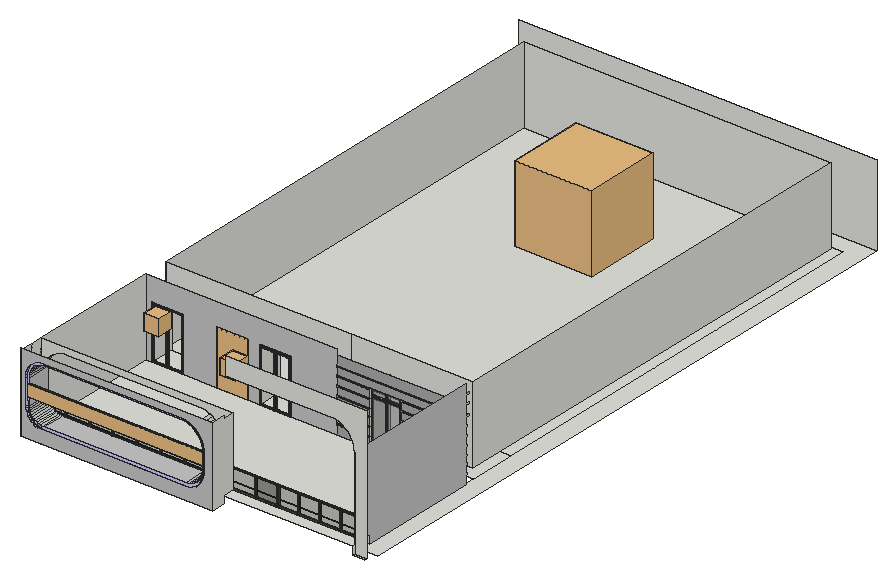
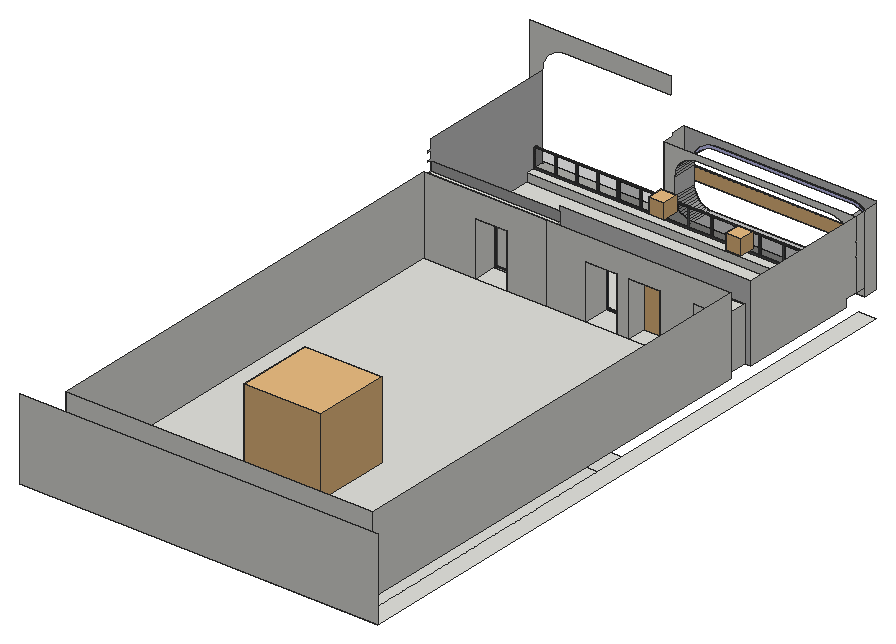
# SketchUp Ruby script. Lengths in inches.
U = 1.inch
M = Sketchup.active_model
def pt(a) = Geom::Point3d.new(a.map { |v| v * U })
def face(e, loops, mat)
  f = e.add_face(loops[0].map { |a| pt(a) })
  loops[1..].each { |l| e.add_face(l.map { |a| pt(a) }).erase! }
  f.material = f.back_material = mat if mat
  f
end
# faces: each face lists its corners as indices into pts; further lists are holes
def faces(e, pts, list, mat = nil) = list.each { |f| face(e, (f[0].is_a?(Array) ? f : [f]).map { |l| l.map { |i| pts[i] } }, mat) }
# xy, xz, yz: faces in a plane at the given z, y or x. An outline is a flat list of corners, or four numbers for a rectangle; further outlines are holes
def ring(l) = l.size == 4 ? [[l[0], l[1]], [l[2], l[1]], [l[2], l[3]], [l[0], l[3]]] : l.each_slice(2).to_a
def flat(e, list, mat, &to3) = list.each { |f| face(e, (f[0].is_a?(Array) ? f : [f]).map { |l| ring(l).map { |u, v| to3.(u, v) } }, mat) }
def xy(e, z, list, mat = nil) = flat(e, list, mat) { |x, y| [x, y, z] }
def xz(e, y, list, mat = nil) = flat(e, list, mat) { |x, z| [x, y, z] }
def yz(e, x, list, mat = nil) = flat(e, list, mat) { |y, z| [x, y, z] }
def lines(e, pts, list) = list.each { |a, b| e.add_line(pt(pts[a]), pt(pts[b])) }
# prism: a flat outline (further loops are holes) pulled along v
def prism(e, loops, v, mat = nil)
  f = face(e, loops, mat); d = Geom::Vector3d.new(v.map { |x| x * U })
  f.pushpull(f.normal.samedirection?(d) ? d.length : -d.length)
end
def box(e, o, s, mat = nil) = prism(e, [[o, [o[0] + s[0], o[1], o[2]], [o[0] + s[0], o[1] + s[1], o[2]], [o[0], o[1] + s[1], o[2]]]], [0, 0, s[2]], mat)
def at(x, y, z, deg = 0) = Geom::Transformation.translation(pt([x, y, z])) * Geom::Transformation.rotation(ORIGIN, Z_AXIS, deg.degrees)
def axes(o, x, y, z) = Geom::Transformation.new([*x, 0, *y, 0, *z, 0, *pt(o).to_a, 1])
def part(name) = M.definitions.add(name)
# library, detail: a bought-in or finely detailed component or shape, given as its bounding box
def library(name, o, s) = part(name).tap { |d| box(d.entities, o, s) }
def detail(e, o, s) = box(e.add_group.entities, o, s)
def put(e, d, t, mat = nil) = e.add_instance(d, t).tap { |i| i.material = mat if mat }
def group(e, t, mat = nil) = e.add_group.tap { |g| g.transformation = t; g.material = mat if mat }.entities
root = M.entities
M.materials.add("Aluminum_Polished").color = [83, 85, 85]
M.materials.add("Glass_Window_Neutral").color = [0, 0, 0]
M.materials["Glass_Window_Neutral"].alpha = 0.125
M.materials.add("Wine2").color = [0, 0, 0]
M.materials["Wine2"].alpha = 0
M.materials.add("[0130_Gainsboro]").color = [39, 45, 50]
M.materials.add("[Color I01]").color = [204, 204, 255]
M.materials.add("[Color M02]").color = [198, 198, 198]
M.materials.add("[Color M03]").color = [170, 170, 170]
M.materials.add("[Color M06]").color = [86, 86, 86]
M.materials.add("[Translucent Glass Gray]").color = [128, 128, 128]
M.materials["[Translucent Glass Gray]"].alpha = 0.5
c1 = part("Framed glazing panel")
xy(c1.entities,0,[[0,-0.98,43.07,0],[0,0,43.07,1.4]],"[0130_Gainsboro]")
xy(c1.entities,0.3,[[0.3,-1.43,42.77,-0.98]],"[0130_Gainsboro]")
xy(c1.entities,2.95,[[2.95,-1.43,40.12,-0.63],[2.95,-0.63,40.12,0],[2.95,0,40.12,0.64],[2.95,0.64,40.12,1.4]],"[0130_Gainsboro]")
xy(c1.entities,3.54,[[3.54,-0.63,39.53,0],[3.54,0,39.53,0.64]],"[0130_Gainsboro]")
xy(c1.entities,111.8125,[[3.54,-0.63,39.53,0],[3.54,0,39.53,0.64]],"[0130_Gainsboro]")
xy(c1.entities,112.4,[[2.95,-1.43,40.12,-0.63],[2.95,-0.63,40.12,0],[2.95,0,40.12,0.64],[2.95,0.64,40.12,1.4]],"[0130_Gainsboro]")
xy(c1.entities,115.05,[[0.3,-1.43,42.77,-0.98]],"[0130_Gainsboro]")
xy(c1.entities,115.35,[[0,-0.98,43.07,0],[0,0,43.07,1.4]],"[0130_Gainsboro]")
xz(c1.entities,-1.43,[[[0.3,0.3,42.77,115.05],[2.95,2.95,40.12,112.4]]],"[0130_Gainsboro]")
xz(c1.entities,-0.98,[[[0,0,43.07,115.35],[0.3,0.3,42.77,115.05]]],"[0130_Gainsboro]")
xz(c1.entities,-0.63,[[[2.95,2.95,40.12,112.4],[3.54,3.54,39.53,111.8125]]],"[0130_Gainsboro]")
xz(c1.entities,0,[[3.54,3.54,39.53,111.8125]],"Wine2")
xz(c1.entities,0,[[[0,0,43.07,115.35],[2.95,2.95,40.12,112.4]],[[2.95,2.95,40.12,112.4],[3.54,3.54,39.53,111.8125]]],"[0130_Gainsboro]")
xz(c1.entities,0.64,[[[2.95,2.95,40.12,112.4],[3.54,3.54,39.53,111.8125]]],"[0130_Gainsboro]")
xz(c1.entities,1.4,[[[0,0,43.07,115.35],[2.95,2.95,40.12,112.4]]],"[0130_Gainsboro]")
yz(c1.entities,0,[[-0.98,0,0,115.35],[0,0,1.4,115.35]],"[0130_Gainsboro]")
yz(c1.entities,0.3,[[-1.43,0.3,-0.98,115.05]],"[0130_Gainsboro]")
yz(c1.entities,2.95,[[-1.43,2.95,-0.63,112.4],[-0.63,2.95,0,112.4],[0,2.95,0.64,112.4],[0.64,2.95,1.4,112.4]],"[0130_Gainsboro]")
yz(c1.entities,3.54,[[-0.63,3.54,0,111.8125],[0,3.54,0.64,111.8125]],"[0130_Gainsboro]")
yz(c1.entities,39.53,[[-0.63,3.54,0,111.8125],[0,3.54,0.64,111.8125]],"[0130_Gainsboro]")
yz(c1.entities,40.12,[[-1.43,2.95,-0.63,112.4],[-0.63,2.95,0,112.4],[0,2.95,0.64,112.4],[0.64,2.95,1.4,112.4]],"[0130_Gainsboro]")
yz(c1.entities,42.77,[[-1.43,0.3,-0.98,115.05]],"[0130_Gainsboro]")
yz(c1.entities,43.07,[[-0.98,0,0,115.35],[0,0,1.4,115.35]],"[0130_Gainsboro]")
c2 = part("Group\#1")
put(c2.entities,c1,axes([45.29,1.43,0],[1.05148,0,0],[0,1,0],[0,0,1]))
put(c2.entities,c1,axes([0,1.43,0],[1.05148,0,0],[0,1,0],[0,0,1]))
c3 = library("door (1)",[38.93,25.48,0],[40,9.94,82.68])
c4 = part("Group\#3")
xy(c4.entities,0,[[0,0,32.48,1.97]])
xy(c4.entities,0.98,[[0.98,0,31.5,0.98],[0.98,0.98,31.5,1.97]])
xy(c4.entities,8.86,[[0.98,0,31.5,0.98],[0.98,0.98,31.5,1.97]])
xy(c4.entities,9.84,[[0,0,32.48,1.97]])
xz(c4.entities,0,[[[0,0,32.48,9.84],[0.98,0.98,31.5,8.86]]])
xz(c4.entities,0.98,[[0.98,0.98,31.5,8.86]],"[Translucent Glass Gray]")
xz(c4.entities,1.97,[[[0,0,32.48,9.84],[0.98,0.98,31.5,8.86]]])
yz(c4.entities,0,[[0,0,1.97,9.84]])
yz(c4.entities,0.98,[[0,0.98,0.98,8.86],[0.98,0.98,1.97,8.86]])
yz(c4.entities,31.5,[[0,0.98,0.98,8.86],[0.98,0.98,1.97,8.86]])
yz(c4.entities,32.48,[[0,0,1.97,9.84]])
c5 = part("Group\#4")
xy(c5.entities,0,[[0,0,32.48,1.97]])
xy(c5.entities,0.98,[[0.98,0,31.5,0.98],[0.98,0.98,31.5,1.97]])
xy(c5.entities,71.85,[[0.98,0,31.5,0.98],[0.98,0.98,31.5,1.97]])
xy(c5.entities,72.83,[[0,0,32.48,1.97]])
xz(c5.entities,0,[[[0,0,32.48,72.83],[0.98,0.98,31.5,71.85]]])
xz(c5.entities,0.98,[[0.98,0.98,31.5,71.85]],"[Translucent Glass Gray]")
xz(c5.entities,1.97,[[[0,0,32.48,72.83],[0.98,0.98,31.5,71.85]]])
yz(c5.entities,0,[[0,0,1.97,72.83]])
yz(c5.entities,0.98,[[0,0.98,0.98,71.85],[0.98,0.98,1.97,71.85]])
yz(c5.entities,31.5,[[0,0.98,0.98,71.85],[0.98,0.98,1.97,71.85]])
yz(c5.entities,32.48,[[0,0,1.97,72.83]])
c6 = part("FIXED+GLASS+WINDOW+WITH+TRANSOM")
g1 = group(c6.entities,at(0,0,0))
xy(g1,0,[[0,0,70.86,3.9375]])
xy(g1,1.97,[[1.97,0,34.45,0.98],[36.42,0,68.9,3.9375],[1.97,2.95,34.45,3.9375]])
xy(g1,86.61,[[1.97,0,34.45,3.9375],[34.45,0,36.42,3.9375],[36.42,0,68.9,3.9375]])
xy(g1,88.58,[[0,0,70.86,3.9375]])
xz(g1,0,[[[0,0,70.86,88.58],[1.97,1.97,34.45,86.61],[36.42,1.97,68.9,86.61]]])
xz(g1,3.9375,[[[0,0,70.86,88.58],[1.97,1.97,34.45,86.61],[36.42,1.97,68.9,86.61]]])
yz(g1,0,[[0,0,3.9375,88.58]])
yz(g1,1.97,[[0,1.97,3.9375,74.8],[0,76.77,3.9375,86.61]])
yz(g1,34.45,[[0,1.97,3.9375,86.61]])
yz(g1,36.42,[[0,1.97,3.9375,86.61]])
yz(g1,68.9,[[0,1.97,3.9375,86.61]])
yz(g1,70.86,[[0,0,3.9375,88.58]])
g2 = group(g1,at(1.97,0,74.8))
box(g2,[0,0,0],[66.93,3.9375,1.97])
put(g1,c4,at(1.97,0.98,76.77))
put(g1,c4,at(36.42,0.98,76.77))
put(g1,c5,at(1.97,0.98,1.97))
put(g1,c5,at(36.42,0.98,1.97))
c7 = library("Omni Light",[-12,-12,-12],[24,24,24])
c8 = part("Group\#54")
box(c8.entities,[0,0,0],[2,1,28])
c9 = part("Group\#56")
p = [[0.11,0.32,0.14],[0.11,0.69,0.14]]
lines(c9.entities,p,[[0,1]])
g3 = group(c9.entities,at(0.11,0,0))
prism(g3,[[[0,0.24,0],[0,0.32,0.14],[0,0.24,0.27],[0,0.08,0.27],[0,0,0.14],[0,0.08,0]]],[-0.11,0,0])
c10 = part("Ver Glass Railing")
g4 = group(c10.entities,at(0,0,0),"Aluminum_Polished")
box(g4,[0,0,0],[2,185,2])
g5 = group(c10.entities,at(0,0,2),"Aluminum_Polished")
p = [[1.41,1,0],[1.41,36.8,0],[1.41,184,0],[1.29,184,0],[1.29,1,0],[1.29,36.8,0],
  [1.41,184,28],[1.29,184,28],[1.41,148.2,28],[1.29,148.2,28],[1.41,1,28],[1.29,1,28],
  [1.29,111.4,28],[1.29,111.4,0],[1.41,111.4,0],[1.41,111.4,28],[1.29,110.4,0],[1.29,110.4,28],
  [1.41,110.4,28],[1.41,110.4,0],[1.29,74.6,28],[1.29,74.6,0],[1.41,74.6,0],[1.41,74.6,28],
  [1.29,73.6,0],[1.29,73.6,28],[1.41,73.6,28],[1.41,73.6,0],[1.29,148.2,0],[1.41,148.2,0],
  [1.29,147.2,0],[1.29,147.2,28],[1.41,147.2,28],[1.41,147.2,0],[1.29,37.8,28],[1.29,37.8,0],
  [1.41,37.8,0],[1.41,37.8,28],[1.29,36.8,28],[1.41,36.8,28]]
lines(g5,p,[[0,1],[2,3],[4,5],[6,7],[6,8],[7,9],[10,11],[2,6],[3,7],[0,4],[11,4],[10,0],
  [12,13],[14,15],[16,17],[18,19],[20,21],[22,23],[24,25],[26,27],[27,22],[24,21],[23,26],[20,25],
  [9,28],[29,8],[30,31],[32,33],[33,29],[30,28],[8,32],[9,31],[34,35],[36,37],[5,38],[39,1],
  [1,36],[5,35],[37,39],[14,33],[19,14],[22,19],[36,27],[13,30],[16,13],[21,16],[35,24],[15,18],
  [12,17],[29,2],[28,3],[18,23],[32,15],[17,20],[31,12],[26,37],[25,34],[34,38],[39,10],[38,11]])
g6 = group(g5,at(1.79,1,0))
box(g6,[-0.5,0,0],[0.125,183,28],"Glass_Window_Neutral")
g7 = group(g5,at(0,184,28))
box(g7,[0,-184,0],[2.5,185,1])
put(g5,c8,axes([2,185,28],[-1,0,0],[0,-1,0],[0,0,-1]))
put(g5,c8,axes([2,1,28],[-1,0,0],[0,-1,0],[0,0,-1]))
put(g5,c8,axes([2,111.4,28],[-1,0,0],[0,-1,0],[0,0,-1]))
put(g5,c8,axes([2,74.6,28],[-1,0,0],[0,-1,0],[0,0,-1]))
g8 = group(g5,at(2,148.2,28))
box(g8,[-2,-1,-28],[2,1,28])
put(g5,c8,axes([2,37.8,28],[-1,0,0],[0,-1,0],[0,0,-1]))
put(g5,c9,at(1.17,146.31,24.26))
put(g5,c9,axes([1.17,148.89,24.54],[1,0,0],[0,-1,0],[0,0,-1]))
put(g5,c9,axes([1.17,148.89,4.79],[1,0,0],[0,-1,0],[0,0,-1]))
put(g5,c9,at(1.17,146.31,4.51))
put(g5,c9,at(1.17,109.51,4.51))
put(g5,c9,axes([1.17,112.09,4.79],[1,0,0],[0,-1,0],[0,0,-1]))
put(g5,c9,axes([1.17,112.09,24.54],[1,0,0],[0,-1,0],[0,0,-1]))
put(g5,c9,at(1.17,109.51,24.26))
put(g5,c9,axes([1.17,75.29,24.54],[1,0,0],[0,-1,0],[0,0,-1]))
put(g5,c9,at(1.17,72.71,4.51))
put(g5,c9,axes([1.17,75.29,4.79],[1,0,0],[0,-1,0],[0,0,-1]))
put(g5,c9,at(1.17,72.71,24.26))
put(g5,c9,axes([1.17,38.49,24.54],[1,0,0],[0,-1,0],[0,0,-1]))
put(g5,c9,at(1.17,35.91,4.51))
put(g5,c9,axes([1.17,38.49,4.79],[1,0,0],[0,-1,0],[0,0,-1]))
put(g5,c9,at(1.17,35.91,24.26))
c11 = library("Mesh Light",[-0.5,-0.5,-0.1],[1,1,0.2])
c12 = library("Omni Light\#3",[-12,-12,-12],[24,24,24])
c13 = library("Omni Light\#4",[-12,-12,-12],[24,24,24])
xy(root,109.25,[[512.63,317.48,510.71,317.74,508.91,318.48,507.375,319.66,506.19,321.2,505.45,323,505.2,324.92,505.45,326.85,506.19,328.64,507.375,330.18,508.91,331.36,510.71,332.1,512.63,332.36,514.56,332.1,516.35,331.36,517.89,330.18,519.07,328.64,519.82,326.85,520.07,324.92,519.82,323,519.07,321.2,517.89,319.66,516.35,318.48,514.56,317.74],[333.76,319.66,332.4,319.84,331.13,320.37,330.04,321.2,329.21,322.29,328.68,323.56,328.5,324.92,328.68,326.28,329.21,327.55,330.04,328.64,331.13,329.47,332.4,330,333.76,330.18,335.12,330,336.39,329.47,337.48,328.64,338.3125,327.55,338.84,326.28,339.02,324.92,338.84,323.56,338.3125,322.29,337.48,321.2,336.39,320.37,335.12,319.84],[137.46,319.67,136.1,319.85,134.84,320.375,133.75,321.21,132.91,322.3,132.39,323.5625,132.21,324.92,132.39,326.28,132.91,327.55,133.75,328.63,134.84,329.47,136.1,329.99,137.46,330.17,138.82,329.99,140.09,329.47,141.17,328.63,142.01,327.55,142.53,326.28,142.71,324.92,142.53,323.5625,142.01,322.3,141.17,321.21,140.09,320.375,138.82,319.85],[221.33,320.11,220.08,320.27,218.92,320.75,217.92,321.52,217.16,322.51,216.68,323.67,216.51,324.92,216.68,326.17,217.16,327.33,217.92,328.32,218.92,329.09,220.08,329.57,221.33,329.73,222.57,329.57,223.73,329.09,224.73,328.32,225.5,327.33,225.98,326.17,226.14,324.92,225.98,323.67,225.5,322.51,224.73,321.52,223.73,320.75,222.57,320.27]])
xy(root,120,[[52.9375,244.9375,52.9375,1217.1875,610.25,1217.1875,610.25,244.9375,582.4,244.9375,582.4,1189.34,80.78,1189.34,80.78,244.9375],[388.8,467.53,388.8,752.85,420.8,752.85,420.8,539.85,582.4,539.85,582.4,467.53],[420.8,539.85,420.8,752.85,80.78,752.85,80.78,1189.34,582.4,1189.34,582.4,539.85],[80.78,706.78,388.8,752.85]])
xy(root,126,[[591.56,219.25,610.25,222.9375],[591.56,253.93,591.56,440.75,489.92,440.75,489.92,479.76,441.92,479.76,441.92,440.75,317.61,440.75,317.61,479.76,269.61,479.76,269.61,440.75,250.74,440.75,250.74,479.76,202.74,479.76,202.74,440.75,149.24,440.75,149.24,479.76,101.24,479.76,101.24,440.75,91.81,440.75,91.81,255],[91.94,479.76,571.24,1178.18]])
xy(root,126.375,[[91.81,197.75,390.47,219.25]])
xy(root,138.5625,[[390.47,219.25,591.56,219.25,591.56,253.93,91.81,255,91.81,237.125,390.47,237.125],[91.81,219.25,390.47,237.125]])
xy(root,140.19,[[390.47,440.75,441.92,442.6875],[489.92,440.75,591.56,442.6875]])
xy(root,142.88,[[390.47,440.75,441.92,442.6875],[489.92,440.75,591.56,442.6875]])
xy(root,148.85,[[125.12,200.3125,346.02,237.125]],"[Color M02]")
xy(root,154.39,[[390.47,440.75,441.92,442.6875],[489.92,440.75,591.56,442.6875]])
xy(root,157.08,[[390.47,440.75,441.92,442.6875],[489.92,440.75,591.56,442.6875]])
xy(root,165.66,[[489.92,440.75,591.56,442.6875]])
xy(root,167.29,[[390.47,440.75,441.92,442.6875]])
xy(root,168.35,[[489.92,440.75,591.56,442.6875]])
xy(root,169.98,[[390.47,440.75,441.92,442.6875]])
xy(root,178.68,[[390.47,440.75,441.92,442.6875]])
xy(root,179.23,[[489.92,440.75,591.56,442.6875]])
xy(root,181.36,[[390.47,440.75,441.92,442.6875]])
xy(root,181.92,[[489.92,440.75,591.56,442.6875]])
xy(root,192.79,[[390.47,440.75,441.92,442.6875],[489.92,440.75,591.56,442.6875]])
xy(root,195.48,[[390.47,440.75,441.92,442.6875],[489.92,440.75,591.56,442.6875]])
xy(root,206.92,[[390.47,440.75,441.92,442.6875],[489.92,440.75,591.56,442.6875]])
xy(root,209.61,[[390.47,440.75,441.92,442.6875],[489.92,440.75,591.56,442.6875]])
xy(root,210,[[101.24,440.75,149.24,479.76],[202.74,440.75,250.74,479.76],[269.61,440.75,317.61,479.76],[441.92,440.75,489.92,479.76]])
xy(root,220.21,[[390.47,440.75,591.56,446.25]])
xy(root,222.9,[[390.47,440.75,591.56,446.25]])
xz(root,197.75,[[[91.81,126.375,390.47,126.375,390.47,249.875,91.94,249.875,91.94,246,91.81,246],[346.02,145.02,125.12,145.85,121.8,146.0625,118.54,146.71,115.39,147.78,112.41,149.25,109.65,151.1,107.15,153.29,104.96,155.79,103.11,158.55,101.64,161.54,100.57,164.69,99.92,167.95,99.7,171.26,98.88,210.57,99.13,214.44,99.89,218.25,101.14,221.92,102.85,225.4,105.01,228.63,107.57,231.55,110.49,234.11,113.71,236.26,117.19,237.98,120.87,239.23,124.68,239.99,339.27,240.24,344.16,239.92,348.98,238.96,353.625,237.38,358.03,235.21,362.11,232.49,365.8,229.25,369.03,225.5625,371.76,221.48,373.93,217.08,375.51,212.43,376.46,207.62,376.79,202.72,376.79,175.78,376.52,171.77,375.74,167.82,374.44,164.01,372.66,160.4,370.43,157.06,367.77,154.03,364.75,151.38,361.4,149.14,357.79,147.36,353.98,146.07,350.04,145.28]]],"[Color M02]")
xz(root,219.25,[[91.81,126.375,390.47,138.5625]])
xz(root,222.9375,[[591.56,126,591.56,267.76,591.24,272.57,590.3,277.3,588.75,281.87,586.62,286.19,583.9375,290.2,580.76,293.83,577.13,297.01,573.12,299.6875,568.79,301.82,564.23,303.37,559.5,304.31,554.68,304.625,390.47,304.625,390.47,331.6875,610.25,331.6875,610.25,126]])
xz(root,237.125,[[[91.81,138.5625,390.47,246],[125.12,148.85,346.02,148.85,349.54,149.08,352.99,149.77,356.33,150.9,359.49,152.46,362.42,154.41,365.07,156.74,367.39,159.39,369.35,162.32,370.91,165.48,372.04,168.8125,372.73,172.27,372.96,175.78,372.96,202.72,372.67,207.12,371.81,211.44,370.39,215.61,368.44,219.57,365.99,223.23,363.09,226.54,359.78,229.45,356.11,231.9,352.16,233.85,347.99,235.26,343.66,236.12,339.27,236.41,128.55,236.41,125.18,236.19,121.86,235.53,118.66,234.44,115.63,232.95,112.82,231.07,110.28,228.84,108.05,226.3,106.17,223.49,104.67,220.46,103.59,217.26,102.93,213.94,102.71,210.57,102.71,171.26,102.9,168.34,103.47,165.46,104.41,162.6875,105.71,160.06,107.34,157.62,109.27,155.41,111.48,153.48,113.91,151.85,116.54,150.55,119.32,149.61,122.2,149.04]]])
xz(root,440.75,[[91.81,126,101.24,126,101.24,210,149.24,210,149.24,126,202.74,126,202.74,210,250.74,210,250.74,126,269.61,126,269.61,210,317.61,210,317.61,126,390.47,126,390.47,246,91.81,246]],"[Color M02]")
xz(root,440.75,[[390.47,126,441.92,140.19],[489.92,126,591.56,140.19],[390.47,142.88,441.92,154.39],[489.92,142.88,591.56,154.39],[390.47,157.08,441.92,167.29],
  [489.92,157.08,591.56,165.66],[489.92,168.35,591.56,179.23],[390.47,169.98,441.92,178.68],[390.47,181.36,441.92,192.79],[489.92,181.92,591.56,192.79],
  [390.47,195.48,441.92,206.92],[489.92,195.48,591.56,206.92],[390.47,209.61,441.92,209.61,441.92,210,489.92,210,489.92,209.61,591.56,209.61,591.56,220.21,390.47,220.21],[390.47,222.9,591.56,237.98]],"[Color M03]")
xz(root,442.6875,[[390.47,140.19,441.92,142.88],[489.92,140.19,591.56,142.88],[390.47,154.39,441.92,157.08],[489.92,154.39,591.56,157.08],[489.92,165.66,591.56,168.35],
  [390.47,167.29,441.92,169.98],[390.47,178.68,441.92,181.36],[489.92,179.23,591.56,181.92],[390.47,192.79,441.92,195.48],[489.92,192.79,591.56,195.48],
  [390.47,206.92,441.92,209.61],[489.92,206.92,591.56,209.61]],"[Color M06]")
xz(root,446.25,[[390.47,220.21,591.56,222.9]],"[Color M06]")
xz(root,479.76,[[91.94,126,91.94,246,381.14,246,381.14,126,317.61,126,317.61,210,269.61,210,269.61,126,250.74,126,250.74,210,202.74,210,202.74,126,149.24,126,149.24,210,101.24,210,101.24,126],[381.14,126,381.14,246,571.24,246,571.24,126,489.92,126,489.92,210,441.92,210,441.92,126]])
xz(root,1178.18,[[91.94,126,571.24,246]])
xz(root,1217.1875,[[52.9375,120,610.25,246]])
yz(root,91.81,[[255,126,440.75,126,440.75,246,237.125,246,237.125,138.5625,255,138.5625],[197.75,126.375,219.25,246],[219.25,138.5625,237.125,246]])
yz(root,91.94,[[479.76,126,1178.18,246]])
yz(root,101.24,[[440.75,126,479.76,210]])
yz(root,102.71,[[200.3125,171.26,237.125,210.57]],"[Color M02]")
yz(root,149.24,[[440.75,126,479.76,210]])
yz(root,202.74,[[440.75,126,479.76,210]])
yz(root,250.74,[[440.75,126,479.76,210]])
yz(root,269.61,[[440.75,126,479.76,210]])
yz(root,317.61,[[440.75,126,479.76,210]])
yz(root,372.96,[[200.3125,175.78,237.125,202.72]],"[Color M02]")
yz(root,376.79,[[197.75,175.78,200.3125,202.72]],"[Color I01]")
yz(root,390.47,[[197.75,126.375,219.25,126.375,219.25,138.5625,237.125,138.5625,237.125,246,219.25,246,219.25,249.875,197.75,249.875],[440.75,140.19,442.6875,142.88],[440.75,154.39,442.6875,157.08],[440.75,167.29,442.6875,169.98],[440.75,178.68,442.6875,181.36],
  [440.75,192.79,442.6875,195.48],[440.75,206.92,442.6875,209.61],[440.75,220.21,446.25,222.9]])
yz(root,441.92,[[440.75,126,479.76,126,479.76,210,440.75,210,440.75,209.61,442.6875,209.61,442.6875,206.92,440.75,206.92,440.75,195.48,442.6875,195.48,442.6875,192.79,440.75,192.79,440.75,181.36,442.6875,181.36,442.6875,178.68,440.75,178.68,440.75,169.98,442.6875,169.98,442.6875,167.29,440.75,167.29,440.75,157.08,442.6875,157.08,442.6875,154.39,440.75,154.39,440.75,142.88,442.6875,142.88,442.6875,140.19,440.75,140.19]])
yz(root,489.92,[[440.75,126,440.75,140.19,442.6875,140.19,442.6875,142.88,440.75,142.88,440.75,154.39,442.6875,154.39,442.6875,157.08,440.75,157.08,440.75,165.66,442.6875,165.66,442.6875,168.35,440.75,168.35,440.75,179.23,442.6875,179.23,442.6875,181.92,440.75,181.92,440.75,192.79,442.6875,192.79,442.6875,195.48,440.75,195.48,440.75,206.92,442.6875,206.92,442.6875,209.61,440.75,209.61,440.75,210,479.76,210,479.76,126]])
yz(root,571.24,[[479.76,126,1178.18,246]])
yz(root,591.56,[[219.25,126,222.9375,138.5625]])
yz(root,591.56,[[253.93,126,253.93,138.5625,222.9375,138.5625,222.9375,267.76,440.75,267.76,440.75,254.07,446.25,254.07,446.25,251.38,440.75,251.38,440.75,240.67,446.25,240.67,446.25,237.98,440.75,237.98,440.75,222.9,446.25,222.9,446.25,220.21,440.75,220.21,440.75,209.61,442.6875,209.61,442.6875,206.92,440.75,206.92,440.75,195.48,442.6875,195.48,442.6875,192.79,440.75,192.79,440.75,181.92,442.6875,181.92,442.6875,179.23,440.75,179.23,440.75,168.35,442.6875,168.35,442.6875,165.66,440.75,165.66,440.75,157.08,442.6875,157.08,442.6875,154.39,440.75,154.39,440.75,142.88,442.6875,142.88,442.6875,140.19,440.75,140.19,440.75,126]],"[Color M02]")
p = [[591.56,253.93,126],[91.81,255,126],[91.81,255,138.5625],[591.56,253.93,138.5625],[125.12,197.75,145.85],[346.02,197.75,145.02],
  [346.02,200.3125,145.02],[125.12,200.3125,145.85],[350.04,197.75,145.28],[350.04,200.3125,145.28],[353.98,197.75,146.07],[353.98,200.3125,146.07],
  [121.8,197.75,146.0625],[121.8,200.3125,146.0625],[357.79,197.75,147.36],[357.79,200.3125,147.36],[118.54,197.75,146.71],[118.54,200.3125,146.71],
  [115.39,197.75,147.78],[115.39,200.3125,147.78],[361.4,197.75,149.14],[361.4,200.3125,149.14],[112.41,197.75,149.25],[112.41,200.3125,149.25],
  [122.2,237.125,149.04],[122.2,200.3125,149.04],[125.12,200.3125,148.85],[125.12,237.125,148.85],[346.02,237.125,148.85],[346.02,200.3125,148.85],
  [349.54,200.3125,149.08],[349.54,237.125,149.08],[119.32,237.125,149.61],[119.32,200.3125,149.61],[364.75,197.75,151.38],[364.75,200.3125,151.38],
  [352.99,200.3125,149.77],[352.99,237.125,149.77],[109.65,197.75,151.1],[109.65,200.3125,151.1],[116.54,237.125,150.55],[116.54,200.3125,150.55],
  [356.33,200.3125,150.9],[356.33,237.125,150.9],[113.91,237.125,151.85],[113.91,200.3125,151.85],[359.49,200.3125,152.46],[359.49,237.125,152.46],
  [107.15,197.75,153.29],[107.15,200.3125,153.29],[367.77,197.75,154.03],[367.77,200.3125,154.03],[111.48,237.125,153.48],[111.48,200.3125,153.48],
  [362.42,200.3125,154.41],[362.42,237.125,154.41],[104.96,197.75,155.79],[104.96,200.3125,155.79],[109.27,237.125,155.41],[109.27,200.3125,155.41],
  [370.43,197.75,157.06],[370.43,200.3125,157.06],[365.07,200.3125,156.74],[365.07,237.125,156.74],[107.34,237.125,157.62],[107.34,200.3125,157.62],
  [103.11,197.75,158.55],[103.11,200.3125,158.55],[367.39,200.3125,159.39],[367.39,237.125,159.39],[372.66,197.75,160.4],[372.66,200.3125,160.4],
  [105.71,237.125,160.06],[105.71,200.3125,160.06],[101.64,197.75,161.54],[101.64,200.3125,161.54],[369.35,200.3125,162.32],[369.35,237.125,162.32],
  [104.41,237.125,162.6875],[104.41,200.3125,162.6875],[374.44,197.75,164.01],[374.44,200.3125,164.01],[100.57,197.75,164.69],[100.57,200.3125,164.69],
  [370.91,200.3125,165.48],[370.91,237.125,165.48],[103.47,237.125,165.46],[103.47,200.3125,165.46],[375.74,197.75,167.82],[375.74,200.3125,167.82],
  [99.92,197.75,167.95],[99.92,200.3125,167.95],[102.9,237.125,168.34],[102.9,200.3125,168.34],[372.04,200.3125,168.8125],[372.04,237.125,168.8125],
  [376.52,197.75,171.77],[376.52,200.3125,171.77],[99.7,197.75,171.26],[99.7,200.3125,171.26],[102.71,237.125,171.26],[102.71,200.3125,171.26],
  [372.73,200.3125,172.27],[372.73,237.125,172.27],[98.88,197.75,210.57],[98.88,200.3125,210.57],[376.79,197.75,175.78],[376.79,200.3125,175.78],
  [372.96,200.3125,175.78],[372.96,237.125,175.78],[376.79,197.75,202.72],[376.46,197.75,207.62],[376.46,200.3125,207.62],[376.79,200.3125,202.72],
  [372.96,237.125,202.72],[372.96,200.3125,202.72],[372.67,200.3125,207.12],[372.67,237.125,207.12],[371.81,200.3125,211.44],[371.81,237.125,211.44],
  [375.51,197.75,212.43],[375.51,200.3125,212.43],[99.13,197.75,214.44],[99.13,200.3125,214.44],[102.93,237.125,213.94],[102.93,200.3125,213.94],
  [102.71,200.3125,210.57],[102.71,237.125,210.57],[370.39,200.3125,215.61],[370.39,237.125,215.61],[373.93,197.75,217.08],[373.93,200.3125,217.08],
  [103.59,237.125,217.26],[103.59,200.3125,217.26],[99.89,197.75,218.25],[99.89,200.3125,218.25],[368.44,200.3125,219.57],[368.44,237.125,219.57],
  [371.76,197.75,221.48],[371.76,200.3125,221.48],[104.67,237.125,220.46],[104.67,200.3125,220.46],[101.14,197.75,221.92],[101.14,200.3125,221.92],
  [365.99,200.3125,223.23],[365.99,237.125,223.23],[106.17,237.125,223.49],[106.17,200.3125,223.49],[369.03,197.75,225.5625],[369.03,200.3125,225.5625],
  [102.85,197.75,225.4],[102.85,200.3125,225.4],[363.09,200.3125,226.54],[363.09,237.125,226.54],[108.05,237.125,226.3],[108.05,200.3125,226.3],
  [105.01,197.75,228.63],[105.01,200.3125,228.63],[365.8,197.75,229.25],[365.8,200.3125,229.25],[110.28,237.125,228.84],[110.28,200.3125,228.84],
  [359.78,200.3125,229.45],[359.78,237.125,229.45],[107.57,197.75,231.55],[107.57,200.3125,231.55],[112.82,237.125,231.07],[112.82,200.3125,231.07],
  [362.11,197.75,232.49],[362.11,200.3125,232.49],[356.11,200.3125,231.9],[356.11,237.125,231.9]]
faces(root,p,[[0,1,2,3]])
faces(root,p,[[4,5,6,7],[5,8,9,6],[8,10,11,9],[12,4,7,13],[10,14,15,11],[16,12,13,17],[18,16,17,19],[14,20,21,15],
  [22,18,19,23],[20,34,35,21],[38,22,23,39],[48,38,39,49],[34,50,51,35],[56,48,49,57],[50,60,61,51],[66,56,57,67],
  [60,70,71,61],[74,66,67,75],[70,80,81,71],[82,74,75,83],[80,88,89,81],[90,82,83,91],[88,96,97,89],[98,90,91,99],
  [104,98,99,105],[96,106,107,97],[110,111,112,113],[111,120,121,112],[122,104,105,123],[120,130,131,121],[134,122,123,135],[130,138,139,131],
  [142,134,135,143],[138,148,149,139],[150,142,143,151],[156,150,151,157],[148,158,159,149],[164,156,157,165],[158,168,169,159]],"[Color I01]")
faces(root,p,[[24,25,26,27],[28,29,30,31],[32,33,25,24],[31,30,36,37],[40,41,33,32],[37,36,42,43],[44,45,41,40],[43,42,46,47],
  [52,53,45,44],[47,46,54,55],[58,59,53,52],[55,54,62,63],[64,65,59,58],[63,62,68,69],[72,73,65,64],[69,68,76,77],
  [78,79,73,72],[77,76,84,85],[86,87,79,78],[92,93,87,86],[85,84,94,95],[100,101,93,92],[95,94,102,103],[103,102,108,109],
  [114,115,116,117],[117,116,118,119],[124,125,126,127],[119,118,128,129],[132,133,125,124],[129,128,136,137],[140,141,133,132],[137,136,144,145],
  [146,147,141,140],[145,144,152,153],[154,155,147,146],[160,161,155,154],[153,152,162,163],[166,167,161,160],[163,162,170,171]],"[Color M02]")
put(root,c2,axes([270.48,440.75,126],[0.52722,0,0],[0,-0.55,0],[0,0,0.72819]))
put(root,c2,axes([101.49,442.31,126],[0.52722,0,0],[0,-0.55,0],[0,0,0.72819]))
put(root,c3,axes([156.03,415.26,126],[1.2,0,0],[0,1,0],[0,0,1.02]))
put(root,c6,axes([441.92,442.09,126],[0.66,0,0],[0,0.66,0],[0,0,0.94827]))
put(root,c7,axes([340.125,984.86,198],[5,0,0],[0,5,0],[0,0,5]))
put(root,c10,at(91.88,239.625,138.5625,-90))
put(root,c10,at(276.88,239.625,138.5625,-90))
put(root,c10,axes([425.76,239.625,138.5625],[0,-1,0],[0.89623,0,0],[0,0,1]))
g9 = group(root,at(98.88,200.3125,145.02))
xz(g9,0,[[[247.14,0,251.16,0.26,255.11,1.05,258.92,2.34,262.52,4.12,265.87,6.36,268.9,9.01,271.55,12.04,273.79,15.38,275.57,18.99,276.86,22.8,277.64,26.75,277.91,30.76,277.91,57.7,277.59,62.6,276.63,67.41,275.05,72.06,272.88,76.46,270.15,80.54,266.92,84.23,263.23,87.47,259.15,90.19,254.75,92.36,250.1,93.94,245.29,94.9,240.39,95.22,25.8,94.97,21.99,94.21,18.32,92.96,14.84,91.24,11.61,89.09,8.69,86.53,6.13,83.61,3.98,80.38,2.26,76.9,1.01,73.23,0.25,69.42,0,65.55,0.83,26.24,1.04,22.93,1.69,19.67,2.76,16.52,4.23,13.53,6.08,10.77,8.27,8.27,10.77,6.08,13.53,4.23,16.52,2.76,19.67,1.69,22.93,1.04,26.24,0.83],[26.24,3.83,23.32,4.02,20.44,4.59,17.67,5.53,15.04,6.83,12.6,8.46,10.39,10.39,8.46,12.6,6.83,15.04,5.53,17.67,4.59,20.44,4.02,23.32,3.83,26.24,3.83,65.55,4.05,68.92,4.71,72.24,5.8,75.4375,7.29,78.47,9.17,81.28,11.4,83.82,13.9375,86.05,16.75,87.93,19.78,89.42,22.98,90.51,26.3,91.17,29.67,91.39,240.39,91.39,244.79,91.1,249.11,90.24,253.28,88.83,257.23,86.88,260.9,84.43,264.21,81.52,267.12,78.21,269.56,74.55,271.51,70.59,272.93,66.42,273.79,62.1,274.08,57.7,274.08,30.76,273.85,27.25,273.16,23.79,272.03,20.46,270.47,17.3,268.51,14.37,266.1875,11.72,263.54,9.39,260.61,7.4375,257.45,5.88,254.11,4.75,250.66,4.06,247.14,3.83]]],"[Color I01]")
put(g9,c11,axes([138.95,0,47.61],[278.90722,0,0],[0,1,0],[0,0,96.21972]))
put(root,c12,at(306.1,345.05,234.95))
put(root,c13,at(170.24,365.23,240.6))
